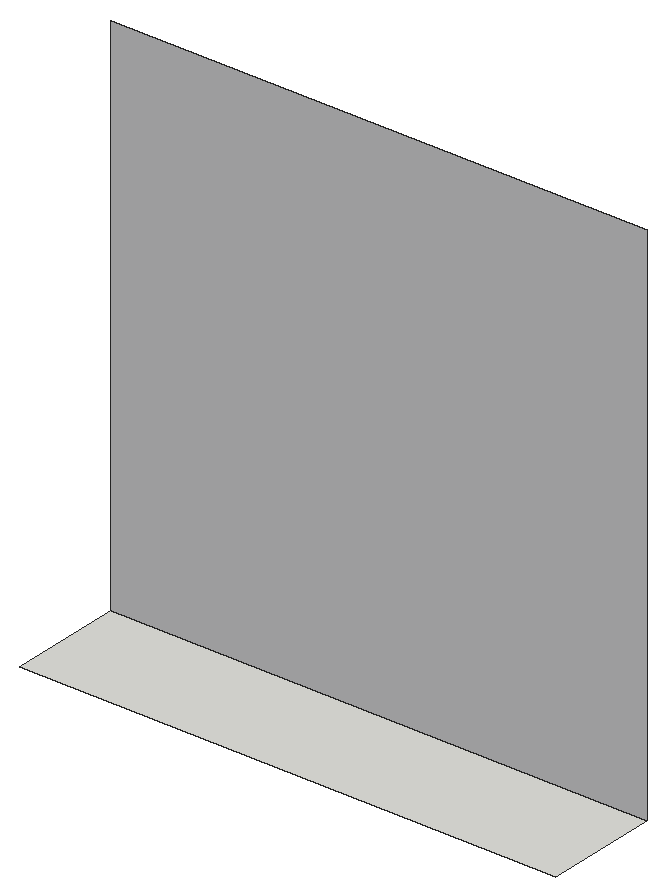
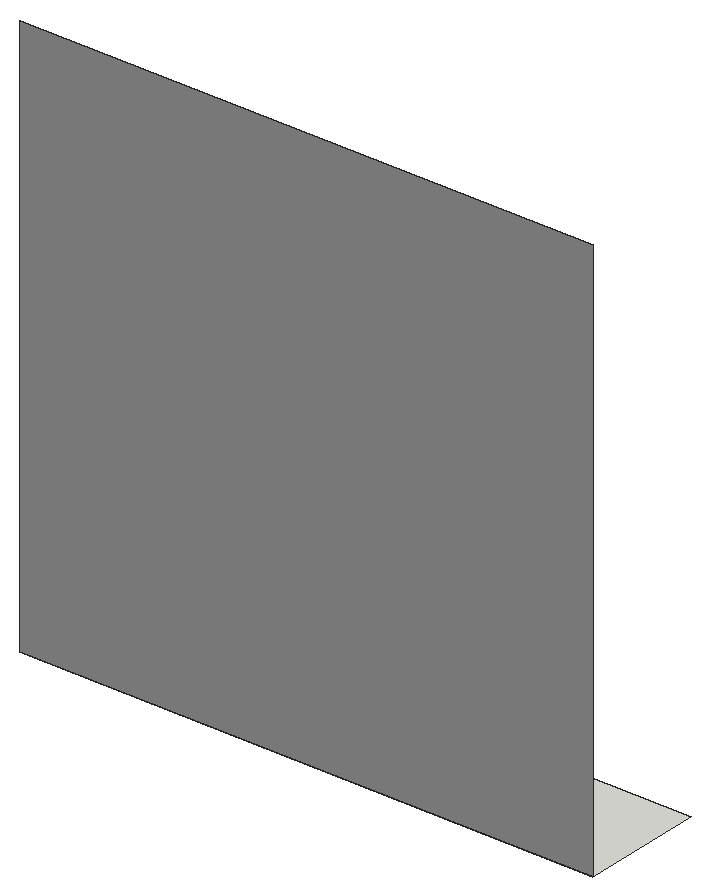
# SketchUp Ruby script. Lengths in inches.
U = 1.inch
M = Sketchup.active_model
def pt(a) = Geom::Point3d.new(a.map { |v| v * U })
def face(e, loops, mat)
  f = e.add_face(loops[0].map { |a| pt(a) })
  loops[1..].each { |l| e.add_face(l.map { |a| pt(a) }).erase! }
  f.material = f.back_material = mat if mat
  f
end
# faces: each face lists its corners as indices into pts; further lists are holes
def faces(e, pts, list, mat = nil) = list.each { |f| face(e, (f[0].is_a?(Array) ? f : [f]).map { |l| l.map { |i| pts[i] } }, mat) }
# xy, xz, yz: faces in a plane at the given z, y or x. An outline is a flat list of corners, or four numbers for a rectangle; further outlines are holes
def ring(l) = l.size == 4 ? [[l[0], l[1]], [l[2], l[1]], [l[2], l[3]], [l[0], l[3]]] : l.each_slice(2).to_a
def flat(e, list, mat, &to3) = list.each { |f| face(e, (f[0].is_a?(Array) ? f : [f]).map { |l| ring(l).map { |u, v| to3.(u, v) } }, mat) }
def xy(e, z, list, mat = nil) = flat(e, list, mat) { |x, y| [x, y, z] }
def xz(e, y, list, mat = nil) = flat(e, list, mat) { |x, z| [x, y, z] }
def yz(e, x, list, mat = nil) = flat(e, list, mat) { |y, z| [x, y, z] }
def lines(e, pts, list) = list.each { |a, b| e.add_line(pt(pts[a]), pt(pts[b])) }
# prism: a flat outline (further loops are holes) pulled along v
def prism(e, loops, v, mat = nil)
  f = face(e, loops, mat); d = Geom::Vector3d.new(v.map { |x| x * U })
  f.pushpull(f.normal.samedirection?(d) ? d.length : -d.length)
end
def box(e, o, s, mat = nil) = prism(e, [[o, [o[0] + s[0], o[1], o[2]], [o[0] + s[0], o[1] + s[1], o[2]], [o[0], o[1] + s[1], o[2]]]], [0, 0, s[2]], mat)
def at(x, y, z, deg = 0) = Geom::Transformation.translation(pt([x, y, z])) * Geom::Transformation.rotation(ORIGIN, Z_AXIS, deg.degrees)
def axes(o, x, y, z) = Geom::Transformation.new([*x, 0, *y, 0, *z, 0, *pt(o).to_a, 1])
def part(name) = M.definitions.add(name)
# library, detail: a bought-in or finely detailed component or shape, given as its bounding box
def library(name, o, s) = part(name).tap { |d| box(d.entities, o, s) }
def detail(e, o, s) = box(e.add_group.entities, o, s)
def put(e, d, t, mat = nil) = e.add_instance(d, t).tap { |i| i.material = mat if mat }
def group(e, t, mat = nil) = e.add_group.tap { |g| g.transformation = t; g.material = mat if mat }.entities
root = M.entities
M.materials.add("[Fencing Metal Straight]").color = [194, 195, 196]
xy(root,17.625,[[14.48,0,113.3,21.02]])
xz(root,21.02,[[14.48,17.625,113.3,115.1875]],"[Fencing Metal Straight]")
